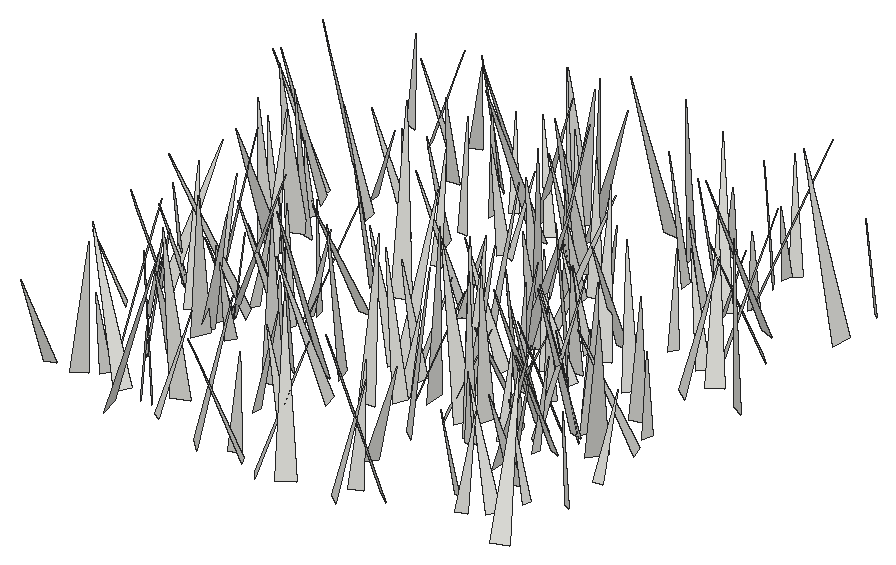
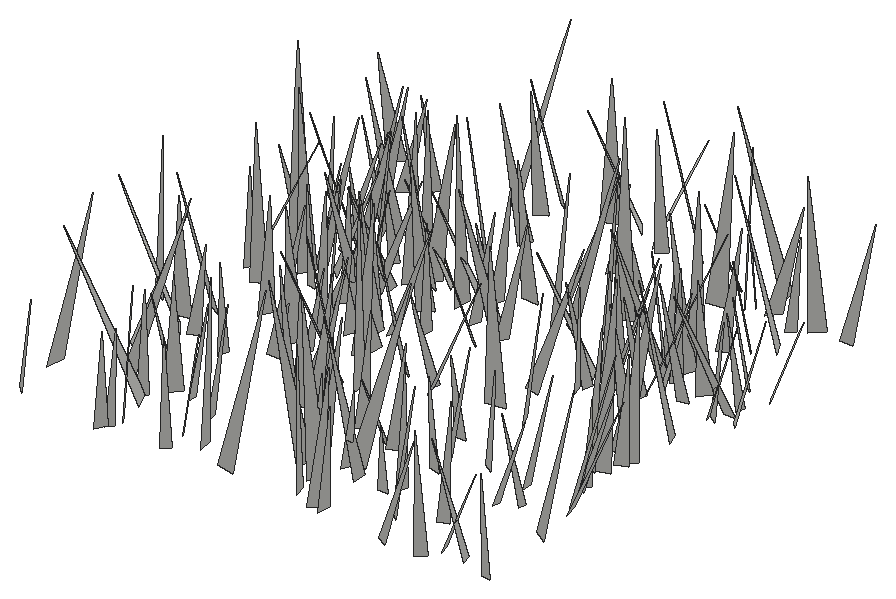
# SketchUp Ruby script. Lengths in inches.
U = 1.inch
M = Sketchup.active_model
def pt(a) = Geom::Point3d.new(a.map { |v| v * U })
def face(e, loops, mat)
  f = e.add_face(loops[0].map { |a| pt(a) })
  loops[1..].each { |l| e.add_face(l.map { |a| pt(a) }).erase! }
  f.material = f.back_material = mat if mat
  f
end
# faces: each face lists its corners as indices into pts; further lists are holes
def faces(e, pts, list, mat = nil) = list.each { |f| face(e, (f[0].is_a?(Array) ? f : [f]).map { |l| l.map { |i| pts[i] } }, mat) }
# xy, xz, yz: faces in a plane at the given z, y or x. An outline is a flat list of corners, or four numbers for a rectangle; further outlines are holes
def ring(l) = l.size == 4 ? [[l[0], l[1]], [l[2], l[1]], [l[2], l[3]], [l[0], l[3]]] : l.each_slice(2).to_a
def flat(e, list, mat, &to3) = list.each { |f| face(e, (f[0].is_a?(Array) ? f : [f]).map { |l| ring(l).map { |u, v| to3.(u, v) } }, mat) }
def xy(e, z, list, mat = nil) = flat(e, list, mat) { |x, y| [x, y, z] }
def xz(e, y, list, mat = nil) = flat(e, list, mat) { |x, z| [x, y, z] }
def yz(e, x, list, mat = nil) = flat(e, list, mat) { |y, z| [x, y, z] }
def lines(e, pts, list) = list.each { |a, b| e.add_line(pt(pts[a]), pt(pts[b])) }
# prism: a flat outline (further loops are holes) pulled along v
def prism(e, loops, v, mat = nil)
  f = face(e, loops, mat); d = Geom::Vector3d.new(v.map { |x| x * U })
  f.pushpull(f.normal.samedirection?(d) ? d.length : -d.length)
end
def box(e, o, s, mat = nil) = prism(e, [[o, [o[0] + s[0], o[1], o[2]], [o[0] + s[0], o[1] + s[1], o[2]], [o[0], o[1] + s[1], o[2]]]], [0, 0, s[2]], mat)
def at(x, y, z, deg = 0) = Geom::Transformation.translation(pt([x, y, z])) * Geom::Transformation.rotation(ORIGIN, Z_AXIS, deg.degrees)
def axes(o, x, y, z) = Geom::Transformation.new([*x, 0, *y, 0, *z, 0, *pt(o).to_a, 1])
def part(name) = M.definitions.add(name)
# library, detail: a bought-in or finely detailed component or shape, given as its bounding box
def library(name, o, s) = part(name).tap { |d| box(d.entities, o, s) }
def detail(e, o, s) = box(e.add_group.entities, o, s)
def put(e, d, t, mat = nil) = e.add_instance(d, t).tap { |i| i.material = mat if mat }
def group(e, t, mat = nil) = e.add_group.tap { |g| g.transformation = t; g.material = mat if mat }.entities
root = M.entities
c1 = part("fur_instance\#9")
p = [[0.8125,0,1.79],[0.67,-0.02,1.48],[0,-0.11,0],[0,0.11,0]]
faces(c1.entities,p,[[0,1,2,3]])
put(root,c1,axes([455.98,342.07,-21.66],[-6.00367,-1.40851,0.07652],[-1.40991,5.98159,-0.51624],[-0.04369,0.52005,6.14503]))
put(root,c1,axes([454.78,319.31,-21.66],[-3.14416,-1.79317,0.28571],[-1.75542,3.14785,0.43854],[0.46429,-0.24163,3.59289]))
put(root,c1,axes([454.56,323.9375,-21.66],[-3.11694,-3.18155,0.61605],[-3.14817,3.17551,0.47138],[0.76862,0.10457,4.42892]))
put(root,c1,axes([455.24,346.7,-21.66],[-3.32824,-5.52708,1.61735],[-5.74671,3.30884,-0.51825],[0.37393,1.65668,6.43096]))
put(root,c1,axes([454.55,354.2,-21.66],[-0.60793,-4.00143,1.69165],[-4.28266,0.83877,0.44495],[0.72934,1.58988,4.02282]))
put(root,c1,axes([456.5625,341.09,-21.66],[-6.28754,-2.52373,1.27093],[-2.51372,6.41179,0.29625],[1.29062,0.19325,6.76865]))
put(root,c1,axes([455.9,308.66,-21.66],[1.11267,-4.69864,0.20362],[-4.67497,-1.12782,-0.47895],[-0.51316,0.0867,4.80478]))
put(root,c1,axes([456.39,324.27,-21.66],[-2.19445,-3.56039,1.55722],[-3.85398,2.22319,-0.34801],[0.4981,1.5159,4.16783]))
put(root,c1,axes([456.87,324.25,-21.66],[-3.51503,-1.89548,0.64915],[-1.82323,3.56963,0.55065],[0.83071,-0.18586,3.95538]))
put(root,c1,axes([457.41,338.99,-21.66],[-2.05359,-3.75931,0.63579],[-3.81243,2.01617,-0.39286],[-0.04503,0.74602,4.26559]))
put(root,c1,axes([455.75,323.04,-21.66],[1.29367,6.30142,0.29631],[6.29029,-1.26564,-0.54746],[0.47747,-0.39942,6.4095]))
put(root,c1,axes([457.38,334.2,-21.66],[1.73924,-4.25815,2.51532],[-4.74882,-2.1825,-0.41111],[-1.38108,2.14207,4.58125]))
put(root,c1,axes([455.6875,321.8,-21.66],[3.70802,-0.97097,0.29213],[-0.94384,-3.70994,-0.3508],[-0.37053,-0.26665,3.81695]))
put(root,c1,axes([457.16,333.47,-21.66],[-4.56803,3.68378,2.77525],[4.20348,4.93276,0.37129],[1.89817,-2.05836,5.85656]))
put(root,c1,axes([457.33,338.51,-21.66],[2.92591,-1.89098,1.19539],[-1.88086,-3.14489,-0.37117],[-1.21125,0.31559,3.46396]))
put(root,c1,axes([457.17,318.95,-21.66],[2.36922,2.94645,1.17355],[3.15581,-2.33594,-0.5062],[-0.31572,-1.23846,3.7468]))
put(root,c1,axes([458.09,335.9,-21.66],[2.83404,-7.21043,2.36501],[-7.48804,-3.06648,-0.37599],[-1.22999,2.05469,7.73827]))
put(root,c1,axes([459.79,352.78,-21.66],[-3.92921,-1.09616,0.24918],[-1.11465,3.91653,-0.34741],[0.14562,0.40197,4.06442]))
put(root,c1,axes([456.86,328.61,-21.66],[6.14666,2.4589,1.36982],[2.59506,-6.2248,-0.47069],[-1.09008,-0.95377,6.60349]))
put(root,c1,axes([459,336.02,-21.66],[1.62899,5.48386,2.82302],[6.01922,-2.05055,0.50999],[-1.34582,-2.53344,5.69792]))
put(root,c1,axes([459.23,321.73,-21.66],[-4.06626,4.25963,1.22614],[4.27905,4.20638,-0.4224],[1.15655,-0.5867,5.87371]))
put(root,c1,axes([458.66,332.7,-21.66],[1.6119,-7.35068,0.1441],[-7.34568,-1.61634,-0.28263],[-0.30696,0.08011,7.52003]))
put(root,c1,axes([457.45,352.96,-21.66],[4.85217,1.44436,0.49792],[1.4914,-4.83766,-0.50049],[-0.33141,-0.62336,5.03778]))
put(root,c1,axes([458.67,308.73,-21.66],[3.92094,-4.8226,1.73149],[-5.06492,-3.97791,0.39007],[-0.77596,1.59628,6.20315]))
put(root,c1,axes([461.06,344.85,-21.66],[-4.01235,0.08097,0.58825],[0.14386,4.03101,0.42638],[0.5761,-0.44265,3.99045]))
put(root,c1,axes([460.87,341.31,-21.66],[-4.89796,-0.50596,1.28828],[-0.38248,5.0478,0.52832],[1.33018,-0.4116,4.8956]))
put(root,c1,axes([460.72,329.2,-21.66],[-0.70792,6.63222,0.94241],[6.69223,0.65809,0.39581],[-0.29764,-0.97786,6.65814]))
put(root,c1,axes([459.9,323.56,-21.66],[-0.06431,5.36711,1.48252],[5.54585,0.19413,-0.46222],[0.49719,-1.47116,5.34755]))
put(root,c1,axes([460.3,309.9,-21.66],[2.53184,-2.74895,1.13947],[-2.76231,-2.72751,-0.44237],[-1.1067,0.51894,3.71097]))
put(root,c1,axes([459.33,343.79,-21.66],[3.75751,0.05108,0.3502],[0.07903,-3.76142,-0.29936],[-0.34497,-0.30538,3.74592]))
put(root,c1,axes([462.99,308.64,-21.66],[-5.62336,3.63446,0.06059],[3.63174,5.6129,0.37548],[-0.15301,-0.3482,6.6851]))
put(root,c1,axes([463.09,323.81,-21.66],[-6.90561,-3.33755,0.10935],[-3.32242,6.89219,0.54573],[0.33571,-0.44394,7.65042]))
put(root,c1,axes([459.26,312.67,-21.66],[6.44327,3.68852,1.42181],[3.82977,-6.4983,-0.49739],[-0.97955,-1.14429,7.40767]))
put(root,c1,axes([460.95,314.05,-21.66],[3.02903,2.92229,1.12241],[2.89072,-3.2105,0.55771],[-1.2014,-0.35704,4.17178]))
put(root,c1,axes([460.53,354.64,-21.66],[2.83156,-3.99697,0.33188],[-4.00855,-2.80696,0.39506],[0.13188,0.49882,4.88236]))
put(root,c1,axes([462.17,323.17,-21.66],[-2.39227,-3.29447,0.41561],[-3.24315,2.42809,0.57931],[0.71291,-0.00928,4.03]))
put(root,c1,axes([462.4,315.54,-21.66],[2.27929,-4.31761,0.37807],[-4.29346,-2.30768,-0.46977],[-0.59235,0.11282,4.85966]))
put(root,c1,axes([462.11,321.53,-21.66],[3.06057,-3.28635,0.3748],[-3.27189,-3.08287,-0.31361],[-0.4851,0.05914,4.47983]))
put(root,c1,axes([462.46,349.53,-21.66],[0.91835,-4.65892,0.5996],[-4.68613,-0.86646,0.44487],[0.32448,0.67241,4.72768]))
put(root,c1,axes([462.28,318.99,-21.66],[5.8288,-3.89293,1.62458],[-3.86791,-6.0381,-0.59132],[-1.68328,0.3943,6.98428]))
put(root,c1,axes([464.28,354.77,-21.66],[-1.9055,-4.08481,0.78377],[-4.15591,1.83492,-0.5407],[-0.16841,0.93717,4.47485]))
put(root,c1,axes([462.74,324.97,-21.66],[4.01633,-1.15722,1.23996],[-1.33038,-4.12648,0.45808],[-1.05202,0.80037,4.15454]))
put(root,c1,axes([462.32,319.71,-21.66],[6.13982,-1.63324,0.91897],[-1.58888,-6.20592,-0.4139],[-0.99371,-0.16841,6.33984]))
put(root,c1,axes([465.27,325.15,-21.66],[-3.54687,-2.63553,0.56126],[-2.61948,3.58991,0.30355],[0.63194,0.08835,4.40842]))
put(root,c1,axes([462.7,322.18,-21.66],[6.72772,1.76518,0.89994],[1.69777,-6.77807,0.60273],[-1.02144,0.36032,6.92927]))
put(root,c1,axes([465.0625,340.8,-21.66],[1.82668,3.73793,1.95155],[3.99067,-2.21946,0.51574],[-1.36206,-1.48974,4.1283]))
put(root,c1,axes([464.49,319.93,-21.66],[2.8154,-3.04723,0.70248],[-2.99803,-2.89898,-0.55973],[-0.88933,0.126,4.11081]))
put(root,c1,axes([466.35,323.77,-21.66],[-5.39834,-1.72938,0.70035],[-1.70183,5.44274,0.32197],[0.76486,-0.09564,5.65943]))
put(root,c1,axes([464.14,320.43,-21.66],[3.95435,2.54343,1.52337],[2.80761,-4.0284,-0.56212],[-0.95239,-1.31514,4.66797]))
put(root,c1,axes([464.8,308.5625,-21.66],[2.81827,1.89164,1.24112],[2.11841,-2.90244,-0.38665],[-0.79437,-1.02901,3.37216]))
put(root,c1,axes([466.09,350.99,-21.66],[-3.7574,-4.18768,1.74578],[-4.4509,3.84178,-0.36412],[0.87968,1.55129,5.61445]))
put(root,c1,axes([465.55,308.93,-21.66],[4.83002,3.67653,3.08875],[4.26917,-5.29337,-0.3752],[-2.19806,-2.20219,6.05848]))
put(root,c1,axes([463.77,305.98,-21.66],[7.81228,1.65656,1.00866],[1.73052,-7.84393,-0.52089],[-0.87571,-0.72239,7.96898]))
put(root,c1,axes([466.83,324.18,-21.66],[-4.7956,1.01448,1.55419],[0.95492,5.04106,-0.34401],[1.59148,0.0322,4.88965]))
put(root,c1,axes([467.27,310.26,-21.66],[-2.10134,6.53759,3.4605],[7.38552,2.05442,0.60354],[0.41142,-3.48856,6.84043]))
put(root,c1,axes([467.3,327.15,-21.66],[-4.422,-0.95671,1.75223],[-1.16644,4.69405,-0.38074],[1.6202,0.76828,4.50826]))
put(root,c1,axes([467.46,333.38,-21.66],[-4.6895,-2.45579,1.69505],[-2.43913,4.97359,0.45768],[1.71894,0.35769,5.27378]))
put(root,c1,axes([467.99,343.6875,-21.66],[0.81104,4.54834,1.26147],[4.65262,-0.98593,0.56355],[-0.7949,-1.13006,4.58559]))
put(root,c1,axes([468.2,341.72,-21.66],[-4.55771,-1.35516,1.4154],[-1.26006,4.77117,0.51063],[1.50069,-0.10962,4.72742]))
put(root,c1,axes([466.92,326.32,-21.66],[4.20297,-1.11156,0.80651],[-1.18233,-4.24977,0.30429],[-0.69867,0.5049,4.33681]))
put(root,c1,axes([467.53,307.08,-21.66],[2.30646,3.84948,0.31393],[3.83736,-2.32546,0.32205],[-0.43787,-0.10267,4.47599]))
put(root,c1,axes([469.01,348.68,-21.66],[-0.87591,3.86506,0.33078],[3.84564,0.82067,0.59405],[-0.50909,-0.4507,3.91829]))
put(root,c1,axes([468.09,347.54,-21.66],[4.81176,-1.3762,1.70282],[-1.26945,-5.10354,-0.53746],[-1.78382,-0.0803,4.97575]))
put(root,c1,axes([467.99,321.15,-21.66],[1.46502,-3.697,0.60293],[-3.73698,-1.39797,0.50827],[0.25762,0.74531,3.94408]))
put(root,c1,axes([469.58,338.58,-21.66],[-0.43977,4.5707,0.64422],[4.59918,0.3789,0.45132],[-0.39225,-0.6818,4.56957]))
put(root,c1,axes([469.91,329.41,-21.66],[-0.6438,-6.00502,0.1729],[-5.98541,0.62626,-0.53591],[-0.51472,0.22839,6.0156]))
put(root,c1,axes([467.79,324.5,-21.66],[5.23362,2.8594,0.35445],[2.818,-5.23298,0.60609],[-0.60055,0.36375,5.93293]))
put(root,c1,axes([470.67,332.96,-21.66],[-1.87564,7.62096,1.95831],[7.8685,1.80971,0.49369],[-0.027,-2.0194,7.83284]))
put(root,c1,axes([470.77,353.71,-21.66],[-4.87312,1.26006,1.29377],[1.19613,5.04128,-0.40455],[1.35309,0.08157,5.01711]))
put(root,c1,axes([470.85,319.28,-21.66],[3.81307,5.29138,3.34018],[5.75803,-4.49829,0.55278],[-2.44962,-2.33704,6.49867]))
put(root,c1,axes([471.57,353.71,-21.66],[3.82096,-4.05561,2.24215],[-4.19487,-4.26194,-0.56033],[-1.96935,1.20949,5.5438]))
put(root,c1,axes([472.53,343.11,-21.66],[-2.40754,3.72637,1.88833],[4.14407,2.40561,0.53634],[0.52762,-1.89079,4.40391]))
put(root,c1,axes([473.53,347.46,-21.66],[-4.1604,2.35856,0.20079],[2.33408,4.15517,-0.44576],[0.39395,0.28953,4.76162]))
put(root,c1,axes([473.5,320.15,-21.66],[-3.27464,-6.78559,1.40651],[-6.92909,3.22889,-0.5548],[0.10135,1.50857,7.51397]))
put(root,c1,axes([471.37,316.39,-21.66],[2.47243,-7.62212,2.09201],[-7.90302,-2.41845,0.52868],[-0.12434,2.1542,7.99563]))
put(root,c1,axes([473.17,346.54,-21.66],[-0.92127,-7.60318,0.93237],[-7.64439,0.85236,-0.60268],[-0.49091,0.99576,7.63504]))
put(root,c1,axes([473.23,342.89,-21.66],[1.4103,3.34023,0.25009],[3.32818,-1.428,0.30438],[-0.37801,-0.11091,3.61295]))
put(root,c1,axes([472.91,312.53,-21.66],[4.24313,0.45781,1.20359],[0.34307,-4.39664,0.46288],[-1.24117,0.34981,4.24258]))
put(root,c1,axes([471.71,348.23,-21.66],[6.64605,0.23955,0.93352],[0.28653,-6.70181,-0.32012],[-0.92019,-0.35664,6.64266]))
put(root,c1,axes([476.02,334.07,-21.66],[-5.88175,-1.50758,0.15009],[-1.51502,5.85044,-0.60606],[-0.00586,0.62434,6.04156]))
put(root,c1,axes([472.59,305.43,-21.66],[4.81614,4.80746,1.57054],[5.00941,-4.83285,-0.56818],[-0.69571,-1.51836,6.78115]))
put(root,c1,axes([474.66,320.8,-21.66],[-6.1633,-1.76581,2.36846],[-1.74431,6.59751,0.37966],[2.38433,0.26209,6.40002]))
put(root,c1,axes([476.3125,317.125,-21.66],[-6.23663,-1.3966,0.55844],[-1.37103,6.25805,0.33911],[0.61857,-0.21031,6.38209]))
put(root,c1,axes([474,352.59,-21.66],[5.47086,1.91538,2.35531],[2.21322,-5.83902,-0.39241],[-2.07794,-1.17628,5.78316]))
put(root,c1,axes([476.96,305.79,-21.66],[-4.6266,-2.97065,0.07987],[-2.96143,4.59663,-0.58091],[-0.24706,0.53178,5.46742]))
put(root,c1,axes([474.44,349.5,-21.66],[0.33482,-6.22736,0.74708],[-6.26175,-0.28913,0.39628],[0.3585,0.76592,6.22375]))
put(root,c1,axes([475.68,348.33,-21.66],[-2.17723,3.86998,1.04919],[4.00343,2.16477,0.32287],[0.22393,-1.07466,4.42864]))
put(root,c1,axes([476.62,324.7,-21.66],[-5.29366,2.0126,1.17564],[2.12712,5.36423,0.39489],[0.95291,-0.79376,5.64955]))
put(root,c1,axes([476.62,311.33,-21.66],[-3.90024,1.94852,0.94584],[2.05782,3.9414,0.36592],[0.67579,-0.75618,4.3445]))
put(root,c1,axes([474.09,350.29,-21.66],[4.71855,-5.46855,1.25045],[-5.59838,-4.69426,0.59612],[-0.35606,1.33873,7.19821]))
put(root,c1,axes([475.66,306.4375,-21.66],[2.40691,-4.24835,1.2679],[-4.42272,-2.4014,0.34948],[-0.30924,1.27831,4.87028]))
put(root,c1,axes([476.49,341.93,-21.66],[3.6689,-2.8215,1.45683],[-2.81207,-3.92099,-0.512],[-1.47496,0.45716,4.59995]))
put(root,c1,axes([476.11,333.45,-21.66],[3.72364,-1.08643,0.80362],[-1.21362,-3.72465,0.58799],[-0.59435,0.79892,3.83407]))
put(root,c1,axes([478.3125,323.32,-21.66],[0.44326,7.59594,0.73525],[7.62112,-0.4789,0.35297],[-0.39679,-0.71255,7.60067]))
put(root,c1,axes([478.82,318.5625,-21.66],[-0.28002,6.79198,1.74012],[7.00527,0.19856,0.35229],[-0.29175,-1.75129,6.78861]))
put(root,c1,axes([476.36,349.05,-21.66],[7.28234,-1.08518,0.65082],[-1.04869,-7.30325,-0.44316],[-0.70811,-0.34428,7.3494]))
put(root,c1,axes([477.91,326.48,-21.66],[2.28219,3.09258,0.57784],[3.14608,-2.24088,-0.43237],[0.01087,-0.72161,3.81909]))
put(root,c1,axes([479.85,323.99,-21.66],[-4.92159,1.07561,1.43405],[1.22896,5.07505,0.41117],[1.30503,-0.72281,5.02095]))
put(root,c1,axes([480.58,320.43,-21.66],[-5.69821,2.17721,0.97614],[2.15034,5.78116,-0.34192],[1.034,-0.02439,6.0904]))
put(root,c1,axes([479.2,344.65,-21.66],[1.80262,-6.00522,1.15434],[-6.08405,-1.88243,-0.2921],[-0.61598,1.01901,6.26312]))
put(root,c1,axes([479.3125,333.05,-21.66],[3.26782,5.25044,1.3347],[5.28581,-3.43164,0.55786],[-1.18691,-0.82697,6.1591]))
put(root,c1,axes([480.54,353.47,-21.66],[-1.04582,-7.4675,1.55674],[-7.62212,0.96116,-0.50998],[-0.30029,1.61039,7.52311]))
put(root,c1,axes([478.87,340.74,-21.66],[-4.56158,-4.36485,4.54967],[-5.17144,5.80258,0.38189],[3.60662,2.79958,6.30192]))
put(root,c1,axes([479.08,304.61,-21.66],[4.55508,3.875,0.43107],[3.83788,-4.57312,0.55448],[-0.68713,0.14532,5.95457]))
put(root,c1,axes([481.54,305.29,-21.66],[-3.76745,6.43232,1.47995],[6.58457,3.78058,0.33053],[0.45645,-1.44608,7.44709]))
put(root,c1,axes([481.69,341.06,-21.66],[-6.39617,-0.72322,1.67284],[-0.5993,6.59982,0.56183],[1.72113,-0.38959,6.41236]))
put(root,c1,axes([480.3,321.28,-21.66],[1.50954,-3.07856,1.78204],[-3.55315,-1.39659,0.59714],[-0.16832,1.87187,3.37633]))
put(root,c1,axes([480.42,337.29,-21.66],[7.19679,1.10507,2.93039],[1.40985,-7.70082,-0.55845],[-2.79655,-1.03845,7.25969]))
put(root,c1,axes([480.7,340.66,-21.66],[-1.22041,-5.00142,1.71972],[-5.19067,1.47111,0.5948],[1.01418,1.51086,5.11369]))
put(root,c1,axes([481.83,327.5,-21.66],[-5.13165,1.21269,1.54361],[1.09048,5.35359,-0.58061],[1.63224,0.23592,5.24093]))
put(root,c1,axes([482.12,342.21,-21.66],[-1.52023,5.3398,1.43684],[5.52962,1.4775,0.35965],[0.03531,-1.48075,5.54032]))
put(root,c1,axes([483.79,329,-21.66],[-5.48132,1.03762,0.48302],[1.07413,5.47965,0.41785],[0.39525,-0.50168,5.563]))
put(root,c1,axes([482.44,322.24,-21.66],[7.55648,0.00384,2.83421],[0.13477,-8.06186,-0.34839],[-2.831,-0.37353,7.54844]))
put(root,c1,axes([481.64,320.82,-21.66],[4.67763,2.46387,0.32375],[2.42875,-4.67875,0.51598],[-0.52599,0.30722,5.26162]))
put(root,c1,axes([484.96,337.22,-21.66],[-3.33504,1.53851,0.16438],[1.54705,3.32218,0.29368],[0.02564,-0.33558,3.66104]))
put(root,c1,axes([483.5,333.28,-21.66],[3.36896,-5.0045,1.18358],[-5.04079,-3.49374,-0.42432],[-1.01802,0.73793,6.01788]))
put(root,c1,axes([484.02,351.55,-21.66],[-6.46976,-1.55499,2.98827],[-1.52534,7.12153,0.40334],[3.00351,0.26714,6.64177]))
put(root,c1,axes([482.45,337.1,-21.66],[3.5807,5.01538,0.32607],[5.01642,-3.54168,-0.61141],[0.30977,-0.61982,6.13202]))
put(root,c1,axes([484.01,324.75,-21.66],[-2.76968,5.79414,2.34049],[6.07448,3.09716,-0.47899],[1.46654,-1.88589,6.4042]))
put(root,c1,axes([484.34,316.76,-21.66],[4.33311,5.30156,2.10924],[5.44411,-4.63436,0.46433],[-1.70794,-1.32191,6.83131]))
put(root,c1,axes([486.43,320.92,-21.66],[5.34271,-3.44394,4.19103],[-3.85612,-6.54857,-0.46545],[-3.8152,1.796,6.33945]))
put(root,c1,axes([486.3,331.11,-21.66],[-4.11869,2.39634,0.55767],[2.352,4.15398,-0.47915],[0.72219,0.13795,4.74094]))
put(root,c1,axes([486.34,348.03,-21.66],[-5.34365,-1.01248,1.41227],[-1.15776,5.47992,-0.452],[1.29585,0.72082,5.4199]))
put(root,c1,axes([483.18,332.08,-21.66],[7.44021,-1.05618,0.97458],[-1.13327,-7.472,0.55406],[-0.88376,0.68976,7.49435]))
put(root,c1,axes([484.74,340.22,-21.66],[4.77554,-0.30271,1.03368],[-0.19329,-4.86277,-0.53104],[-1.0596,-0.47722,4.75556]))
put(root,c1,axes([484.78,329.57,-21.66],[5.5976,-0.64404,1.05715],[-0.59203,-5.69245,-0.3332],[-1.08713,-0.21617,5.62467]))
put(root,c1,axes([486.54,351.14,-21.66],[-3.36264,-2.39418,1.21792],[-2.41208,3.55006,0.31902],[1.18208,0.43333,4.11555]))
put(root,c1,axes([484.59,311.85,-21.66],[4.6953,-3.04636,0.27903],[-3.0591,-4.67738,0.40996],[-0.01004,0.49581,5.58194]))
put(root,c1,axes([487.07,335.24,-21.66],[-3.6032,0.74818,1.09352],[0.87855,3.72087,0.34907],[0.99182,-0.57787,3.66346]))
put(root,c1,axes([486.46,307.64,-21.66],[-2.20726,4.7722,2.01563],[5.04733,2.47451,-0.33147],[1.16667,-1.67676,5.24748]))
put(root,c1,axes([484.77,320.63,-21.66],[4.2362,2.18763,0.04516],[2.18011,-4.21144,-0.49393],[0.18673,-0.4595,4.74206]))
put(root,c1,axes([486.12,321.46,-21.66],[3.51282,6.48869,2.15536],[6.79895,-3.57131,-0.32959],[-0.72316,-2.057,7.37118]))
put(root,c1,axes([486.6,327.5,-21.66],[0.02782,-4.7345,1.86898],[-5.06027,0.17616,0.52158],[0.54982,1.86087,4.70577]))
put(root,c1,axes([486.0625,305.48,-21.66],[3.37327,4.28522,1.21914],[4.44713,-3.33099,-0.5966],[-0.2692,-1.33033,5.4209]))
put(root,c1,axes([486.1875,353.72,-21.66],[1.68114,-3.92704,0.2758],[-3.91607,-1.63754,0.5539],[0.40264,0.46985,4.23569]))
put(root,c1,axes([489.18,330.66,-21.66],[-3.99444,1.28958,0.25526],[1.31279,3.95594,0.55757],[0.06915,-0.60932,4.16025]))
put(root,c1,axes([488.72,308.13,-21.66],[-4.98525,-6.36904,1.05647],[-6.36247,5.07321,0.56124],[1.09531,0.48105,8.06861]))
put(root,c1,axes([488.49,326.92,-21.66],[-4.19066,-2.50752,1.09961],[-2.47633,4.32875,0.43379],[1.16817,0.18082,4.86427]))
put(root,c1,axes([487.59,322.1,-21.66],[6.10585,-2.9623,2.45846],[-2.96929,-6.55789,-0.52733],[-2.45002,0.56525,6.76598]))
put(root,c1,axes([488.67,330.87,-21.66],[-5.61783,-2.93903,2.21928],[-3.25584,5.85535,-0.48739],[1.72124,1.48327,6.32142]))
put(root,c1,axes([488.71,334.77,-21.66],[-4.66477,5.25581,1.41142],[5.28211,4.8201,-0.49149],[1.30953,-0.72026,7.01013]))
put(root,c1,axes([488.82,324.59,-21.66],[-1.13114,-4.608,0.05517],[-4.59723,1.12439,-0.34274],[-0.31976,0.13515,4.73241]))
put(root,c1,axes([488.53,318.93,-21.66],[1.00735,6.64791,2.58508],[7.07427,-1.26504,0.49655],[-0.91221,-2.46923,6.70544]))
put(root,c1,axes([488.2,332.26,-21.66],[1.13187,-5.42392,1.09616],[-5.52646,-1.05128,0.50466],[0.2806,1.17367,5.51773]))
put(root,c1,axes([488.7,337.48,-21.66],[-0.42981,-6.03201,0.26249],[-6.01913,0.44871,0.45551],[0.47339,0.22867,6.03012]))
put(root,c1,axes([489.37,346.49,-21.66],[-3.854,-0.48704,1.31581],[-0.33639,4.05498,0.51565],[1.36213,-0.37663,3.85028]))
put(root,c1,axes([488.74,318.47,-21.66],[-0.48959,-3.44443,1.08487],[-3.54488,0.6673,0.51889],[0.68909,0.98557,3.44014]))
put(root,c1,axes([491.16,346.5,-21.66],[-5.19034,4.80556,0.45379],[4.78626,5.21014,-0.43029],[0.62529,0.00866,7.0603]))
put(root,c1,axes([490.65,322.5625,-21.66],[-6.07164,-2.28107,2.04855],[-2.55827,6.27412,-0.5961],[1.68971,1.3026,6.45854]))
put(root,c1,axes([488.09,323.625,-21.66],[4.49912,0.07902,0.02983],[0.07502,-4.46879,0.52292],[-0.03881,0.52233,4.46932]))
put(root,c1,axes([489.5,327.54,-21.66],[-3.20699,2.34244,2.63387],[2.95903,3.72406,0.29089],[1.91533,-1.83124,3.96071]))
put(root,c1,axes([490.47,320.49,-21.66],[-2.63101,2.88231,1.12737],[2.88894,2.81797,-0.46255],[1.11028,-0.50218,3.87505]))
put(root,c1,axes([491.45,324.09,-21.66],[-1.56855,-7.63886,0.47282],[-7.63369,1.59619,0.46371],[0.55001,0.36889,7.78444]))
put(root,c1,axes([492.02,354.35,-21.66],[-4.07522,2.66076,1.05763],[2.66001,4.19896,-0.31421],[1.05952,-0.30776,4.85678]))
put(root,c1,axes([491.48,352.23,-21.66],[-4.27511,-3.26782,2.05551],[-3.38668,4.64678,0.34365],[1.85313,0.95347,5.37002]))
put(root,c1,axes([492.99,324.52,-21.66],[-3.34237,-3.67886,0.49489],[-3.71061,3.29315,-0.58039],[-0.10119,0.75599,4.93646]))
put(root,c1,axes([491.87,339.58,-21.66],[3.56835,-1.26097,2.05366],[-1.59686,-3.9854,0.32755],[-1.80488,1.03305,3.77039]))
put(root,c1,axes([491.6,353.71,-21.66],[3.2467,-2.02133,0.75684],[-1.94033,-3.33216,-0.57574],[-0.94537,-0.10279,3.78092]))
put(root,c1,axes([493.25,332.6,-21.66],[-5.08391,3.17186,1.29588],[3.17676,5.23223,-0.34381],[1.28383,-0.38638,5.98237]))
put(root,c1,axes([493.02,311.81,-21.66],[-1.62958,-3.15436,1.09529],[-3.33909,1.53504,-0.54711],[-0.01197,1.22427,3.50802]))
put(root,c1,axes([491.64,345.79,-21.66],[3.71055,0.76796,0.33165],[0.80764,-3.68168,-0.51076],[-0.21789,-0.56867,3.7546]))
put(root,c1,axes([492.66,348.41,-21.66],[3.43508,-2.31671,0.74566],[-2.27877,-3.51457,-0.42176],[-0.85461,0.05948,4.12177]))
put(root,c1,axes([494.3,324.62,-21.66],[-2.38494,-6.16406,1.52656],[-6.35023,2.30898,-0.59758],[-0.0234,1.63919,6.58229]))
put(root,c1,axes([493.15,327.25,-21.66],[-0.92871,-3.83483,1.6083],[-4.04735,1.2119,0.55253],[0.95473,1.40727,3.90681]))
put(root,c1,axes([492.6,321.75,-21.66],[4.44163,5.80553,0.93246],[5.82565,-4.50337,0.28854],[-0.79717,-0.56325,7.30404]))
put(root,c1,axes([494.71,321.5625,-21.66],[-1.89303,-4.40404,0.51291],[-4.43222,1.86471,-0.34716],[-0.11875,0.60786,4.78107]))
put(root,c1,axes([493.5625,320.6875,-21.66],[3.9323,-0.29865,1.47953],[-0.48436,-4.16008,0.44758],[-1.42954,0.58799,3.91814]))
put(root,c1,axes([494.91,324.15,-21.66],[-3.3946,-3.12525,1.18102],[-3.29173,3.41661,-0.4203],[0.5714,1.11577,4.59499]))
put(root,c1,axes([495.49,338.6875,-21.66],[-2.79772,3.91125,0.86225],[4.00509,2.73873,0.57209],[0.02536,-1.03446,4.77471]))
put(root,c1,axes([495.8,346.1,-21.66],[-3.1075,-6.9448,0.74353],[-6.98342,3.07514,-0.46373],[-0.12218,0.86773,7.5942]))
put(root,c1,axes([494.07,317.18,-21.66],[4.8135,2.02359,1.54657],[1.94555,-5.05552,0.55956],[-1.64367,-0.05793,5.19149]))
put(root,c1,axes([492.67,317.19,-21.66],[6.50661,-0.43072,0.76621],[-0.39332,-6.54513,-0.33931],[-0.78607,-0.29036,6.51202]))
put(root,c1,axes([492.23,349.07,-21.66],[7.40183,3.33475,0.3809],[3.31775,-7.40888,0.39208],[-0.5081,0.20159,8.10888]))
put(root,c1,axes([496.92,311.35,-21.66],[-4.22119,3.06488,0.48562],[3.10212,4.18863,0.52921],[0.07866,-0.71394,5.1896]))
put(root,c1,axes([495.02,309.83,-21.66],[2.53545,-3.02814,1.98338],[-3.53036,-2.60371,0.53779],[-0.80002,1.89288,3.91266]))
put(root,c1,axes([495.66,315.79,-21.66],[1.37303,-5.10418,0.31363],[-5.09334,-1.39399,-0.38851],[-0.45708,0.20095,5.27134]))
put(root,c1,axes([494.86,325.63,-21.66],[6.65936,-3.07974,1.86174],[-3.09449,-6.89952,-0.34452],[-1.83712,0.458,7.32893]))
put(root,c1,axes([497.94,314.15,-21.66],[-4.0966,0.35691,0.30901],[0.31396,4.07547,-0.54495],[0.35257,0.51784,4.07585]))
put(root,c1,axes([498,336.97,-21.66],[-2.69969,6.39263,0.77147],[6.43614,2.65406,0.5304],[-0.19237,-0.91623,6.91901]))
put(root,c1,axes([498.0625,342.92,-21.66],[-4.1053,-4.23157,0.31859],[-4.21802,4.11764,0.33835],[0.46467,-0.00766,5.88602]))
put(root,c1,axes([499.53,325.53,-21.66],[-5.35424,-1.86738,0.02315],[-1.86377,5.3475,0.29345],[0.11847,-0.26947,5.66294]))
put(root,c1,axes([496.68,329.26,-21.66],[2.3512,-5.85332,1.44977],[-6.03015,-2.28819,0.5412],[-0.02311,1.54732,6.28463]))
put(root,c1,axes([496.62,334.68,-21.66],[3.4607,5.10853,1.2476],[5.25066,-3.43918,-0.48234],[-0.29016,-1.30574,6.15149]))
put(root,c1,axes([496.96,338.55,-21.66],[5.77926,4.78065,0.80242],[4.74367,-5.8345,0.5954],[-0.99801,-0.04845,7.47663]))
put(root,c1,axes([498.79,327.78,-21.66],[3.6892,-1.49713,1.29137],[-1.47127,-3.90506,-0.32413],[-1.32076,0.16824,3.96818]))
put(root,c1,axes([500.32,307.87,-21.66],[-3.69849,5.78351,0.10997],[5.76561,3.69627,-0.48502],[0.46777,0.16892,6.84781]))
put(root,c1,axes([501.01,348.64,-21.66],[-8.03417,0.61584,1.78735],[0.70083,8.21761,0.3188],[1.75577,-0.4621,8.05143]))
put(root,c1,axes([497.5625,323.16,-21.66],[5.80631,-5.6916,0.53269],[-5.68589,-5.82856,-0.29992],[-0.59055,0.15799,8.12513]))
put(root,c1,axes([500.46,353.46,-21.66],[-2.70575,-2.79772,1.42447],[-3.05403,2.78134,-0.3384],[0.7275,1.27058,3.87735]))
put(root,c1,axes([500.65,315.59,-21.66],[1.66971,3.21733,1.57549],[3.35444,-2.01427,0.55833],[-1.25742,-1.10127,3.58153]))
put(root,c1,axes([500.26,319.9375,-21.66],[-0.72601,3.76819,0.7458],[3.80081,0.81458,-0.41575],[0.55615,-0.64789,3.8149]))
put(root,c1,axes([501.49,335.35,-21.66],[-3.98091,-5.38333,3.048],[-6.04161,4.16252,-0.53901],[1.33021,2.79489,6.67363]))
